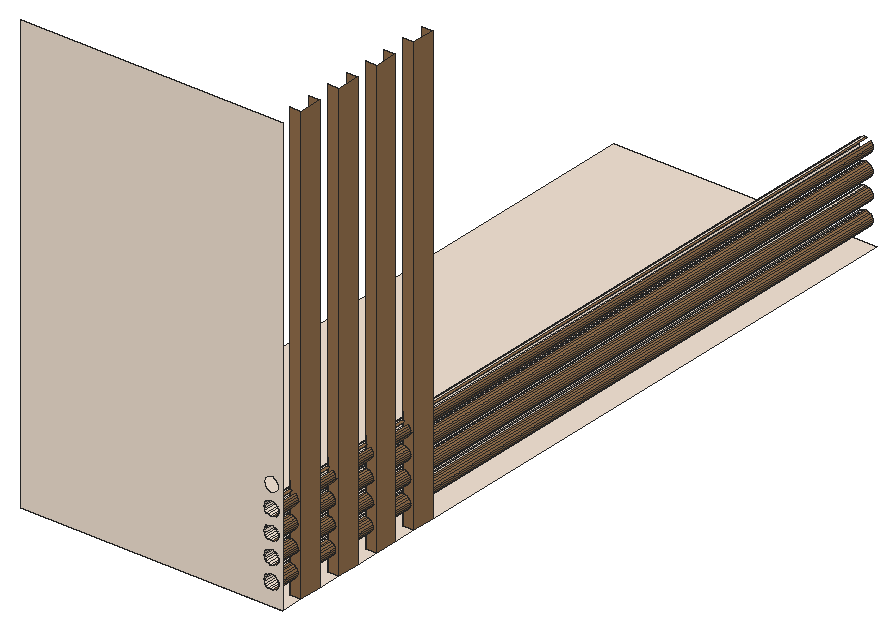
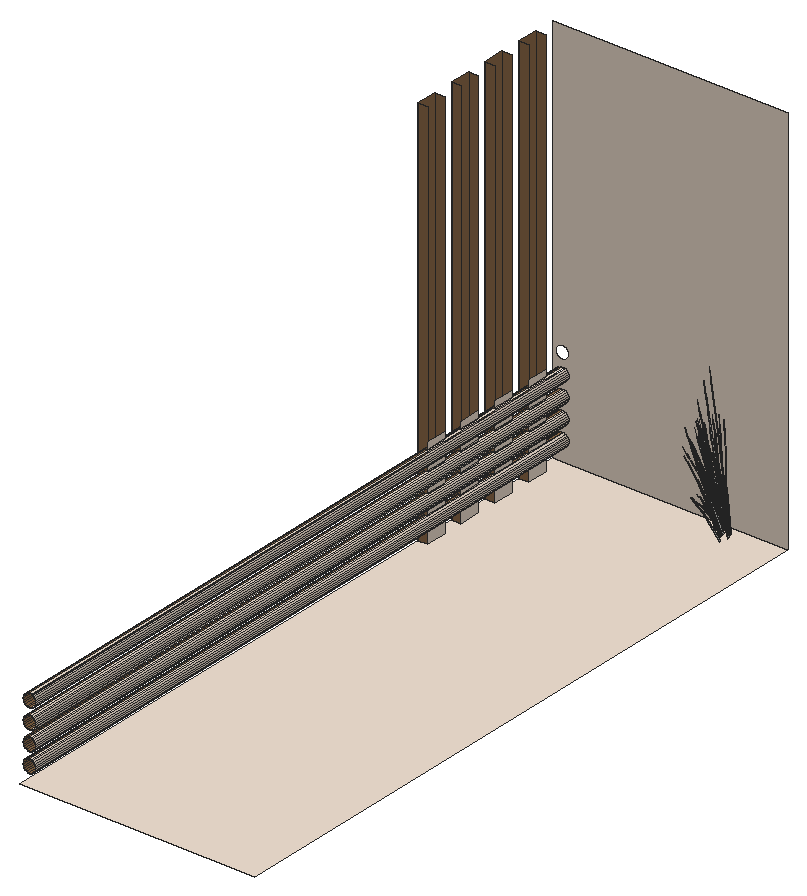
# SketchUp Ruby script. Lengths in inches.
U = 1.inch
M = Sketchup.active_model
def pt(a) = Geom::Point3d.new(a.map { |v| v * U })
def face(e, loops, mat)
  f = e.add_face(loops[0].map { |a| pt(a) })
  loops[1..].each { |l| e.add_face(l.map { |a| pt(a) }).erase! }
  f.material = f.back_material = mat if mat
  f
end
# faces: each face lists its corners as indices into pts; further lists are holes
def faces(e, pts, list, mat = nil) = list.each { |f| face(e, (f[0].is_a?(Array) ? f : [f]).map { |l| l.map { |i| pts[i] } }, mat) }
# xy, xz, yz: faces in a plane at the given z, y or x. An outline is a flat list of corners, or four numbers for a rectangle; further outlines are holes
def ring(l) = l.size == 4 ? [[l[0], l[1]], [l[2], l[1]], [l[2], l[3]], [l[0], l[3]]] : l.each_slice(2).to_a
def flat(e, list, mat, &to3) = list.each { |f| face(e, (f[0].is_a?(Array) ? f : [f]).map { |l| ring(l).map { |u, v| to3.(u, v) } }, mat) }
def xy(e, z, list, mat = nil) = flat(e, list, mat) { |x, y| [x, y, z] }
def xz(e, y, list, mat = nil) = flat(e, list, mat) { |x, z| [x, y, z] }
def yz(e, x, list, mat = nil) = flat(e, list, mat) { |y, z| [x, y, z] }
def lines(e, pts, list) = list.each { |a, b| e.add_line(pt(pts[a]), pt(pts[b])) }
# prism: a flat outline (further loops are holes) pulled along v
def prism(e, loops, v, mat = nil)
  f = face(e, loops, mat); d = Geom::Vector3d.new(v.map { |x| x * U })
  f.pushpull(f.normal.samedirection?(d) ? d.length : -d.length)
end
def box(e, o, s, mat = nil) = prism(e, [[o, [o[0] + s[0], o[1], o[2]], [o[0] + s[0], o[1] + s[1], o[2]], [o[0], o[1] + s[1], o[2]]]], [0, 0, s[2]], mat)
def at(x, y, z, deg = 0) = Geom::Transformation.translation(pt([x, y, z])) * Geom::Transformation.rotation(ORIGIN, Z_AXIS, deg.degrees)
def axes(o, x, y, z) = Geom::Transformation.new([*x, 0, *y, 0, *z, 0, *pt(o).to_a, 1])
def part(name) = M.definitions.add(name)
# library, detail: a bought-in or finely detailed component or shape, given as its bounding box
def library(name, o, s) = part(name).tap { |d| box(d.entities, o, s) }
def detail(e, o, s) = box(e.add_group.entities, o, s)
def put(e, d, t, mat = nil) = e.add_instance(d, t).tap { |i| i.material = mat if mat }
def group(e, t, mat = nil) = e.add_group.tap { |g| g.transformation = t; g.material = mat if mat }.entities
root = M.entities
M.materials.add("C01_Vanilla_Cream").color = [244, 228, 212]
M.materials.add("LightPink_Translucent").color = [144, 107, 117]
M.materials["LightPink_Translucent"].alpha = 0.75
M.materials.add("Wood_Floor_01_1K").color = [146, 111, 76]
c1 = part("blade")
p = [[2.15,0.21,22],[0,0.17,0],[0.09,0.45,0],[2.18,0.31,22],[2.29,0.31,22],[0.38,0.45,0],
  [2.48,0.24,33],[2.49,0.24,33],[2.48,0.22,33]]
faces(c1.entities,p,[[0,1,2,3],[4,5,2,3],[6,3,4,7],[8,0,3,6]])
c2 = part("seeds")
p = [[0.3,-0.1,1.38],[-0.01,-0.03,1.59],[-0.01,-0.03,0.03],[0.14,-0.07,-0.07],[0.29,-0.03,3],[0.15,0.01,3.11]]
faces(c2.entities,p,[[0,1,2,3],[1,0,4,5]],"LightPink_Translucent")
c3 = part("blade with seeds")
put(c3.entities,c1,at(0,0,0))
put(c3.entities,c2,axes([2.4,0.25,30.99],[1.5799,-0.05474,1.17369],[-0.12525,1.92788,0.29478],[-0.07173,-0.02425,1.56792]))
xy(root,462,[[288,12,360,12,360,18.46,357,18.46,357,24.91,360,24.91,360,31.37,357,31.37,357,37.83,360,37.83,360,44.28,357,44.28,357,50.74,360,50.74,360,57.2,357,57.2,357,63.65,360,63.65,360,216,288,216],[357,18.46,360,24.91],[357,31.37,360,37.83],[357,44.28,360,50.74],[357,57.2,360,63.65]],"C01_Vanilla_Cream")
xz(root,12,[[[288,462,360,582],[357,484,357.52,484.07,358,484.27,358.41,484.59,358.73,485,358.93,485.48,359,486,358.93,486.52,358.73,487,358.41,487.41,358,487.73,357.52,487.93,357,488,356.48,487.93,356,487.73,355.59,487.41,355.27,487,355.07,486.52,355,486,355.07,485.48,355.27,485,355.59,484.59,356,484.27,356.48,484.07],[357,490,357.52,490.07,358,490.27,358.41,490.59,358.73,491,358.93,491.48,359,492,358.93,492.52,358.73,493,358.41,493.41,358,493.73,357.52,493.93,357,494,356.48,493.93,356,493.73,355.59,493.41,355.27,493,355.07,492.52,355,492,355.07,491.48,355.27,491,355.59,490.59,356,490.27,356.48,490.07],[357,478,357.52,478.07,358,478.27,358.41,478.59,358.73,479,358.93,479.48,359,480,358.93,480.52,358.73,481,358.41,481.41,358,481.73,357.52,481.93,357,482,356.48,481.93,356,481.73,355.59,481.41,355.27,481,355.07,480.52,355,480,355.07,479.48,355.27,479,355.59,478.59,356,478.27,356.48,478.07],[357,472,357.52,472.07,358,472.27,358.41,472.59,358.73,473,358.93,473.48,359,474,358.93,474.52,358.73,475,358.41,475.41,358,475.73,357.52,475.93,357,476,356.48,475.93,356,475.73,355.59,475.41,355.27,475,355.07,474.52,355,474,355.07,473.48,355.27,473,355.59,472.59,356,472.27,356.48,472.07],[357,466,357.52,466.07,358,466.27,358.41,466.59,358.73,467,358.93,467.48,359,468,358.93,468.52,358.73,469,358.41,469.41,358,469.73,357.52,469.93,357,470,356.48,469.93,356,469.73,355.59,469.41,355.27,469,355.07,468.52,355,468,355.07,467.48,355.27,467,355.59,466.59,356,466.27,356.48,466.07]]],"C01_Vanilla_Cream")
xz(root,18.46,[[357,462,360,582]],"Wood_Floor_01_1K")
xz(root,24.91,[[357,462,360,582]],"Wood_Floor_01_1K")
xz(root,31.37,[[357,462,360,582]],"Wood_Floor_01_1K")
xz(root,37.83,[[357,462,360,582]],"Wood_Floor_01_1K")
xz(root,44.28,[[357,462,360,582]],"Wood_Floor_01_1K")
xz(root,50.74,[[357,462,360,582]],"Wood_Floor_01_1K")
xz(root,57.2,[[357,462,360,582]],"Wood_Floor_01_1K")
xz(root,63.65,[[357,462,360,582]],"Wood_Floor_01_1K")
yz(root,357,[[18.46,462,24.91,466],[31.37,462,37.83,466],[44.28,462,50.74,466],[57.2,462,63.65,466],[18.46,466,24.91,470],
  [31.37,466,37.83,470],[44.28,466,50.74,470],[57.2,466,63.65,470],[18.46,470,24.91,472],[31.37,470,37.83,472],
  [44.28,470,50.74,472],[57.2,470,63.65,472],[18.46,472,24.91,476],[31.37,472,37.83,476],[44.28,472,50.74,476],
  [57.2,472,63.65,476],[18.46,476,24.91,478],[31.37,476,37.83,478],[44.28,476,50.74,478],[57.2,476,63.65,478],
  [18.46,478,24.91,482],[31.37,478,37.83,482],[44.28,478,50.74,482],[57.2,478,63.65,482],[18.46,482,24.91,484],
  [31.37,482,37.83,484],[44.28,482,50.74,484],[57.2,482,63.65,484],[18.46,484,24.91,488],[31.37,484,37.83,488],
  [44.28,484,50.74,488],[57.2,484,63.65,488],[18.46,488,24.91,490],[31.37,488,37.83,490],[44.28,488,50.74,490],
  [57.2,488,63.65,490]],"C01_Vanilla_Cream")
yz(root,360,[[18.46,462,24.91,582],[31.37,462,37.83,582],[44.28,462,50.74,582],[57.2,462,63.65,582]],"Wood_Floor_01_1K")
p = [[356.48,216,466.07],[357,216,466],[357,63.65,466],[357,57.2,466],[357,50.74,466],[357,44.28,466],
  [357,37.83,466],[357,31.37,466],[357,24.91,466],[357,18.46,466],[357,12,466],[356.48,12,466.07],
  [357.52,216,466.07],[357.52,12,466.07],[356,216,466.27],[356,12,466.27],[358,216,466.27],[358,12,466.27],
  [355.59,216,466.59],[355.59,12,466.59],[358.41,216,466.59],[358.41,12,466.59],[355.27,216,467],[355.27,12,467],
  [358.73,216,467],[358.73,12,467],[355.07,216,467.48],[355.07,12,467.48],[358.93,216,467.48],[358.93,12,467.48],
  [355,216,468],[355,12,468],[359,216,468],[359,12,468],[355.07,216,468.52],[355.07,12,468.52],
  [358.93,216,468.52],[358.93,12,468.52],[355.27,216,469],[355.27,12,469],[358.73,216,469],[358.73,12,469],
  [355.59,216,469.41],[355.59,12,469.41],[358.41,216,469.41],[358.41,12,469.41],[356,216,469.73],[356,12,469.73],
  [358,216,469.73],[358,12,469.73],[356.48,216,469.93],[356.48,12,469.93],[357.52,216,469.93],[357.52,12,469.93],
  [357,216,470],[357,12,470],[357,18.46,470],[357,24.91,470],[357,31.37,470],[357,37.83,470],
  [357,44.28,470],[357,50.74,470],[357,57.2,470],[357,63.65,470],[356.48,216,472.07],[357,216,472],
  [357,63.65,472],[357,57.2,472],[357,50.74,472],[357,44.28,472],[357,37.83,472],[357,31.37,472],
  [357,24.91,472],[357,18.46,472],[357,12,472],[356.48,12,472.07],[357.52,216,472.07],[357.52,12,472.07],
  [356,216,472.27],[356,12,472.27],[358,216,472.27],[358,12,472.27],[355.59,216,472.59],[355.59,12,472.59],
  [358.41,216,472.59],[358.41,12,472.59],[355.27,216,473],[355.27,12,473],[358.73,216,473],[358.73,12,473],
  [355.07,216,473.48],[355.07,12,473.48],[358.93,216,473.48],[358.93,12,473.48],[355,216,474],[355,12,474],
  [359,216,474],[359,12,474],[355.07,216,474.52],[355.07,12,474.52],[358.93,216,474.52],[358.93,12,474.52],
  [355.27,216,475],[355.27,12,475],[358.73,216,475],[358.73,12,475],[355.59,216,475.41],[355.59,12,475.41],
  [358.41,216,475.41],[358.41,12,475.41],[356,216,475.73],[356,12,475.73],[358,216,475.73],[358,12,475.73],
  [356.48,216,475.93],[356.48,12,475.93],[357.52,216,475.93],[357.52,12,475.93],[357,216,476],[357,12,476],
  [357,18.46,476],[357,24.91,476],[357,31.37,476],[357,37.83,476],[357,44.28,476],[357,50.74,476],
  [357,57.2,476],[357,63.65,476],[356.48,216,478.07],[357,216,478],[357,63.65,478],[357,57.2,478],
  [357,50.74,478],[357,44.28,478],[357,37.83,478],[357,31.37,478],[357,24.91,478],[357,18.46,478],
  [357,12,478],[356.48,12,478.07],[357.52,216,478.07],[357.52,12,478.07],[356,216,478.27],[356,12,478.27],
  [358,216,478.27],[358,12,478.27],[355.59,216,478.59],[355.59,12,478.59],[358.41,216,478.59],[358.41,12,478.59],
  [355.27,216,479],[355.27,12,479],[358.73,216,479],[358.73,12,479],[355.07,216,479.48],[355.07,12,479.48],
  [358.93,216,479.48],[358.93,12,479.48],[355,216,480],[355,12,480],[359,216,480],[359,12,480],
  [355.07,216,480.52],[355.07,12,480.52],[358.93,216,480.52],[358.93,12,480.52],[355.27,216,481],[355.27,12,481],
  [358.73,216,481],[358.73,12,481],[355.59,216,481.41],[355.59,12,481.41],[358.41,216,481.41],[358.41,12,481.41],
  [356,216,481.73],[356,12,481.73],[358,216,481.73],[358,12,481.73],[356.48,216,481.93],[356.48,12,481.93],
  [357.52,216,481.93],[357.52,12,481.93],[357,216,482],[357,12,482],[357,18.46,482],[357,24.91,482],
  [357,31.37,482],[357,37.83,482],[357,44.28,482],[357,50.74,482],[357,57.2,482],[357,63.65,482],
  [356.48,216,484.07],[357,216,484],[357,63.65,484],[357,57.2,484],[357,50.74,484],[357,44.28,484],
  [357,37.83,484],[357,31.37,484],[357,24.91,484],[357,18.46,484],[357,12,484],[356.48,12,484.07],
  [357.52,216,484.07],[357.52,12,484.07],[356,216,484.27],[356,12,484.27],[358,216,484.27],[358,12,484.27],
  [355.59,216,484.59],[355.59,12,484.59],[358.41,216,484.59],[358.41,12,484.59],[355.27,216,485],[355.27,12,485],
  [358.73,216,485],[358.73,12,485],[355.07,216,485.48],[355.07,12,485.48],[358.93,216,485.48],[358.93,12,485.48],
  [355,216,486],[355,12,486],[359,216,486],[359,12,486],[355.07,216,486.52],[355.07,12,486.52],
  [358.93,216,486.52],[358.93,12,486.52],[355.27,216,487],[355.27,12,487],[358.73,216,487],[358.73,12,487],
  [355.59,216,487.41],[355.59,12,487.41],[358.41,216,487.41],[358.41,12,487.41],[356,216,487.73],[356,12,487.73],
  [357,216,488],[356.48,216,487.93],[356.48,12,487.93],[357,12,488],[357,18.46,488],[357,24.91,488],
  [357,31.37,488],[357,37.83,488],[357,44.28,488],[357,50.74,488],[357,57.2,488],[357,63.65,488],
  [357.52,216,487.93],[357.52,12,487.93]]
faces(root,p,[[0,1,2,3,4,5,6,7,8,9,10,11],[14,0,11,15],[18,14,15,19],[22,18,19,23],[26,22,23,27],[30,26,27,31],[34,30,31,35],[38,34,35,39],
  [42,38,39,43],[46,42,43,47],[50,46,47,51],[54,50,51,55,56,57,58,59,60,61,62,63],[64,65,66,67,68,69,70,71,72,73,74,75],[78,64,75,79],[82,78,79,83],[86,82,83,87],
  [90,86,87,91],[94,90,91,95],[98,94,95,99],[102,98,99,103],[106,102,103,107],[110,106,107,111],[114,110,111,115],[118,114,115,119,120,121,122,123,124,125,126,127],
  [128,129,130,131,132,133,134,135,136,137,138,139],[142,128,139,143],[146,142,143,147],[150,146,147,151],[154,150,151,155],[158,154,155,159],[162,158,159,163],[166,162,163,167],
  [170,166,167,171],[174,170,171,175],[178,174,175,179],[182,178,179,183,184,185,186,187,188,189,190,191],[192,193,194,195,196,197,198,199,200,201,202,203],[206,192,203,207],[210,206,207,211],[214,210,211,215],
  [218,214,215,219],[222,218,219,223],[226,222,223,227],[230,226,227,231],[234,230,231,235],[238,234,235,239],[240,241,242,243,244,245,246,247,248,249,250,251]],"C01_Vanilla_Cream")
faces(root,p,[[1,12,13,10,9,8,7,6,5,4,3,2],[12,16,17,13],[16,20,21,17],[20,24,25,21],[24,28,29,25],[28,32,33,29],[32,36,37,33],[36,40,41,37],
  [40,44,45,41],[44,48,49,45],[48,52,53,49],[52,54,63,62,61,60,59,58,57,56,55,53],[65,76,77,74,73,72,71,70,69,68,67,66],[76,80,81,77],[80,84,85,81],[84,88,89,85],
  [88,92,93,89],[92,96,97,93],[96,100,101,97],[100,104,105,101],[104,108,109,105],[108,112,113,109],[112,116,117,113],[116,118,127,126,125,124,123,122,121,120,119,117],
  [129,140,141,138,137,136,135,134,133,132,131,130],[140,144,145,141],[144,148,149,145],[148,152,153,149],[152,156,157,153],[156,160,161,157],[160,164,165,161],[164,168,169,165],
  [168,172,173,169],[172,176,177,173],[176,180,181,177],[180,182,191,190,189,188,187,186,185,184,183,181],[193,204,205,202,201,200,199,198,197,196,195,194],[204,208,209,205],[208,212,213,209],[212,216,217,213],
  [216,220,221,217],[220,224,225,221],[224,228,229,225],[228,232,233,229],[232,236,237,233],[252,240,251,250,249,248,247,246,245,244,243,253]],"Wood_Floor_01_1K")
put(root,c3,axes([297.43,24.76,468.69],[0.54938,-0.11711,-0.38324],[0.0961,0.44351,-0.29685],[0.14756,0.1271,0.7333]))
put(root,c3,axes([297.93,21.29,466.96],[0.34808,-0.49367,0],[0.58235,0.27531,-0.38706],[0.13264,0.0627,1.22783]))
put(root,c3,axes([298.51,21.08,466.3],[-0.08333,-0.03881,1.32257],[-0.21404,-0.4336,-0.20205],[0.14439,-0.11767,0.22528]))
put(root,c3,axes([298.06,24.23,468.97],[-0.31678,-0.30846,0.2656],[0.36171,-0.29199,-0.3429],[0.18378,0.04443,0.65611]))
put(root,c3,axes([298.25,21.59,466.69],[0.52105,0.24633,-0.37238],[-0.31144,0.44171,0],[0.11867,0.0561,1.18128]))
put(root,c3,axes([298.34,24.51,468.73],[-0.02803,0.37463,0.04823],[-0.42332,-0.01027,0.37966],[0.16216,0.0392,0.57892]))
put(root,c3,axes([298.22,25.09,466.3],[0.04056,-0.07113,1.32257],[0.51066,-0.20948,-0.20205],[0.15482,0.10842,0.22528]))
put(root,c3,axes([298.38,24.39,468.73],[-0.41051,0.32462,0.36002],[-0.35404,-0.34474,0.29685],[0.1926,0.05988,0.74497]))
put(root,c3,axes([298.5,22.12,468.69],[-0.14302,-0.44985,-0.38324],[0.54163,-0.07869,-0.29685],[0.15522,-0.12083,0.7333]))
put(root,c3,axes([299.45,24.44,468.13],[-0.10656,-0.41414,-0.02619],[0.50364,-0.09521,-0.11874],[0.10517,0.02626,0.39164]))
put(root,c3,axes([298.58,23.37,468.97],[-0.46269,-0.13744,0.2656],[0.13495,-0.40096,-0.3429],[0.18628,-0.03677,0.65611]))
put(root,c3,axes([297.49,22.53,466.73],[0.57914,0.08077,-0.46765],[-0.12221,0.49823,-0.12274],[0.17283,0.06037,1.03225]))
put(root,c3,axes([299.95,22.83,466.88],[-0.34516,-0.31503,-0.04866],[0.37803,-0.28865,-0.22062],[0.10711,-0.02032,0.72768]))
put(root,c3,axes([299.16,21.22,467.26],[-0.18544,0.25079,0.86145],[-0.15939,-0.33694,0.63294],[0.15316,-0.08443,0.18974]))
put(root,c3,axes([298.94,22.34,468.73],[0.3822,0.20719,0.04823],[-0.22252,0.29505,0.37966],[0.12254,-0.09539,0.57892]))
put(root,c3,axes([298.83,22.25,468.73],[0.13808,0.45342,0.36002],[-0.54163,0.07869,0.29685],[0.15963,-0.10664,0.74497]))
put(root,c3,axes([297.37,23.6,468.09],[-0.2068,-0.08488,1.28532],[0.42797,-0.35609,0.10393],[0.26673,0.16064,0.54946]))
put(root,c3,axes([300.02,22.32,468.71],[-0.07272,-0.00374,1.33037],[-0.30197,-0.40092,-0.12571],[0.12127,-0.13182,0.23543]))
put(root,c3,axes([298.9,22.17,468.58],[0.48462,-0.07041,-0.2656],[0.12797,0.4025,0.3429],[0.13888,-0.10811,0.65611]))
put(root,c3,axes([298.51,22.3,468.92],[0.29081,-0.38873,-0.53284],[0.5096,0.27626,0.0643],[0.17364,-0.14084,0.75375]))
put(root,c3,axes([299,23.49,468.73],[0.20448,0.33592,0.04823],[-0.37288,0.16442,0.37966],[0.16437,-0.03244,0.57892]))
put(root,c3,axes([298.51,24.39,468.58],[0.31678,0.30846,-0.2656],[-0.36171,0.29199,0.3429],[0.18378,0.04443,0.65611]))
put(root,c3,axes([298.14,24.43,468.96],[0.02981,-0.50103,-0.0912],[0.56442,0.01369,-0.50621],[0.21738,0.0348,0.76918]))
put(root,c3,axes([298.77,23.5,468.96],[-0.28012,-0.44611,-0.0912],[0.49717,-0.21923,-0.50621],[0.20951,-0.05886,0.76918]))
put(root,c3,axes([298.96,23.37,468.73],[-0.15729,0.44921,0.36002],[-0.51712,-0.15361,0.29685],[0.20336,-0.027,0.74497]))
put(root,c3,axes([298.63,24.125,468.72],[0.11943,-0.00833,1.31208],[0.32759,-0.38275,-0.2075],[0.21244,0.05052,0.10523]))
put(root,c3,axes([298.75,23.12,468.69],[0.15083,-0.44814,-0.38324],[0.51712,0.15361,-0.29685],[0.2082,-0.04109,0.7333]))
put(root,c3,axes([300.05,23.4,467.26],[-0.34399,0.08133,0.86145],[0.16192,-0.33614,0.63294],[0.18249,0.023,0.18974]))
put(root,c3,axes([298.93,21.94,467.125],[-0.19889,-0.01459,1.07251],[-0.20376,-0.39145,-0.23066],[0.24434,-0.11074,0.45856]))
put(root,c3,axes([299.07,23.32,468.58],[0.46269,0.13744,-0.2656],[-0.13495,0.40096,0.3429],[0.18628,-0.03677,0.65611]))
put(root,c3,axes([298.17,24.1875,468.92],[0.55654,0.01186,-0.53284],[-0.03738,0.49951,0.0643],[0.23578,0.05271,0.75375]))
put(root,c3,axes([299.3,23.24,466.67],[-0.35858,0.05912,1.06187],[-0.05708,-0.47061,0.06078],[0.25115,-0.07123,0.60425]))
put(root,c3,axes([299.69,22.9375,466.3],[-0.0291,-0.0748,1.32257],[0.20181,-0.43752,-0.20205],[0.20357,-0.00629,0.22528]))
put(root,c3,axes([299.89,24.83,468.71],[-0.05034,-0.04313,1.33037],[0.11012,-0.46232,-0.12571],[0.1983,-0.02954,0.23543]))
put(root,c3,axes([297.8,22.83,468.09],[-0.23093,0.01116,1.28532],[0.15319,-0.4836,0.10393],[0.32909,0.02991,0.54946]))
put(root,c3,axes([298.65,23.28,468.92],[0.48922,-0.21758,-0.53284],[0.27264,0.44789,0.0643],[0.23638,-0.05088,0.75375]))
put(root,c3,axes([300.29,22.8,468.72],[0.07726,-0.07504,1.31208],[-0.09888,-0.46032,-0.2075],[0.19384,-0.08728,0.10523]))
put(root,c3,axes([299.4,23.94,467.125],[-0.13408,-0.12117,1.07251],[0.17446,-0.40083,-0.23066],[0.27128,0.0543,0.45856]))
